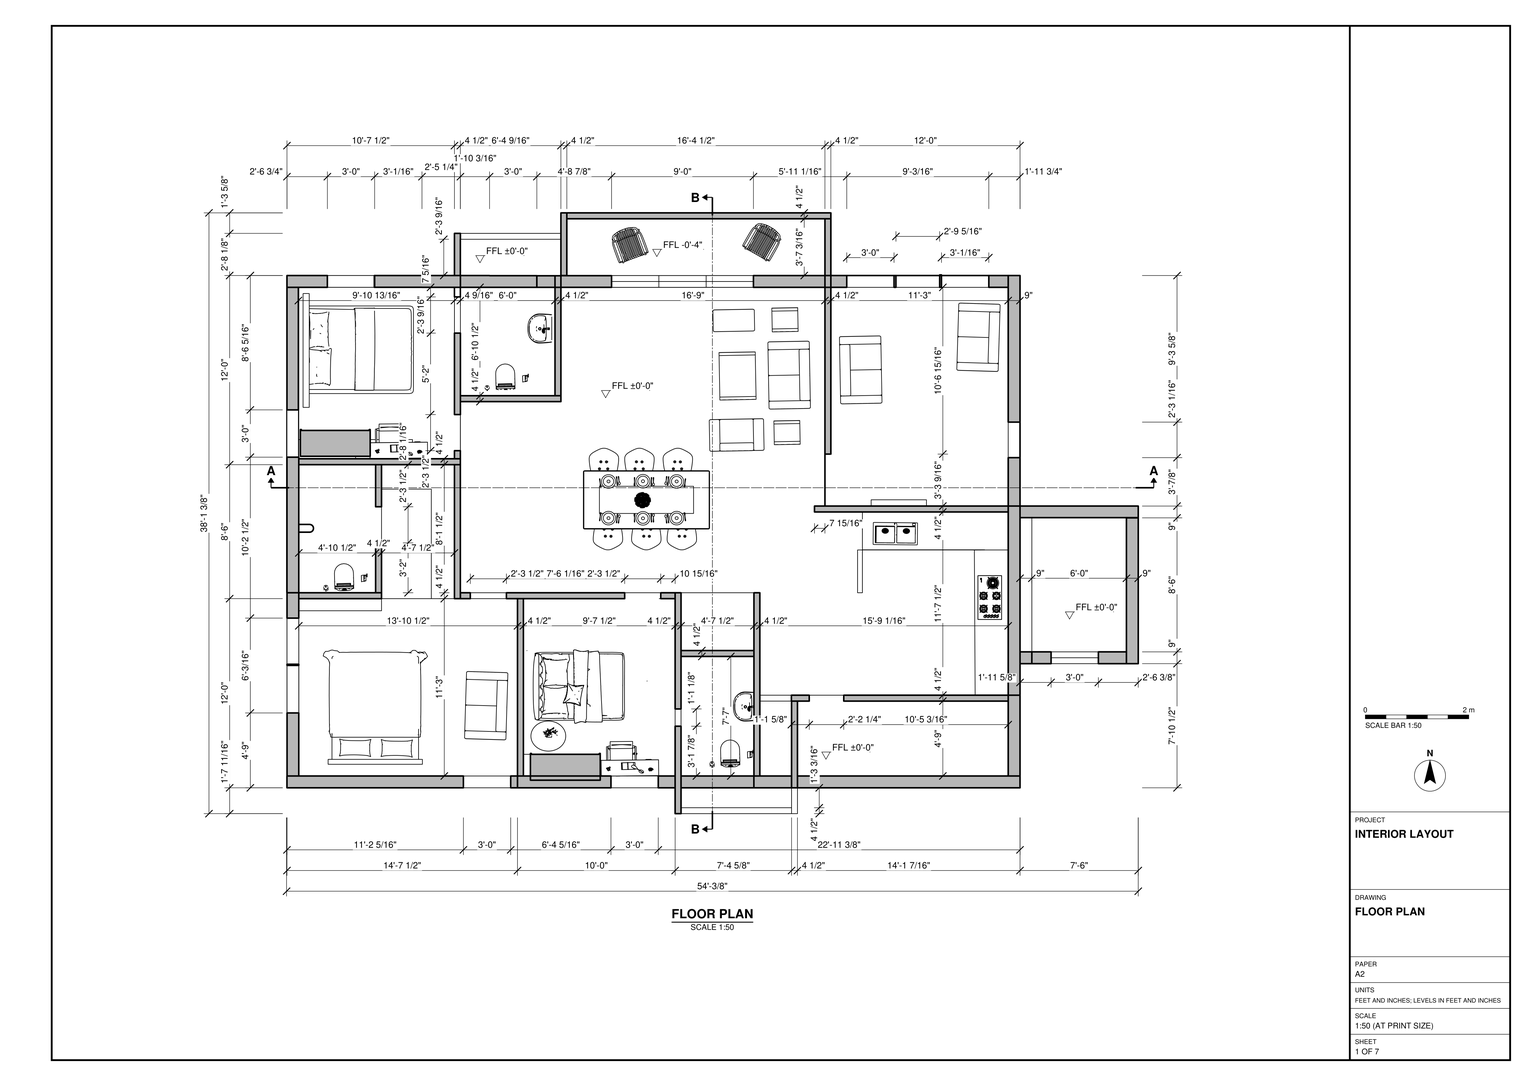
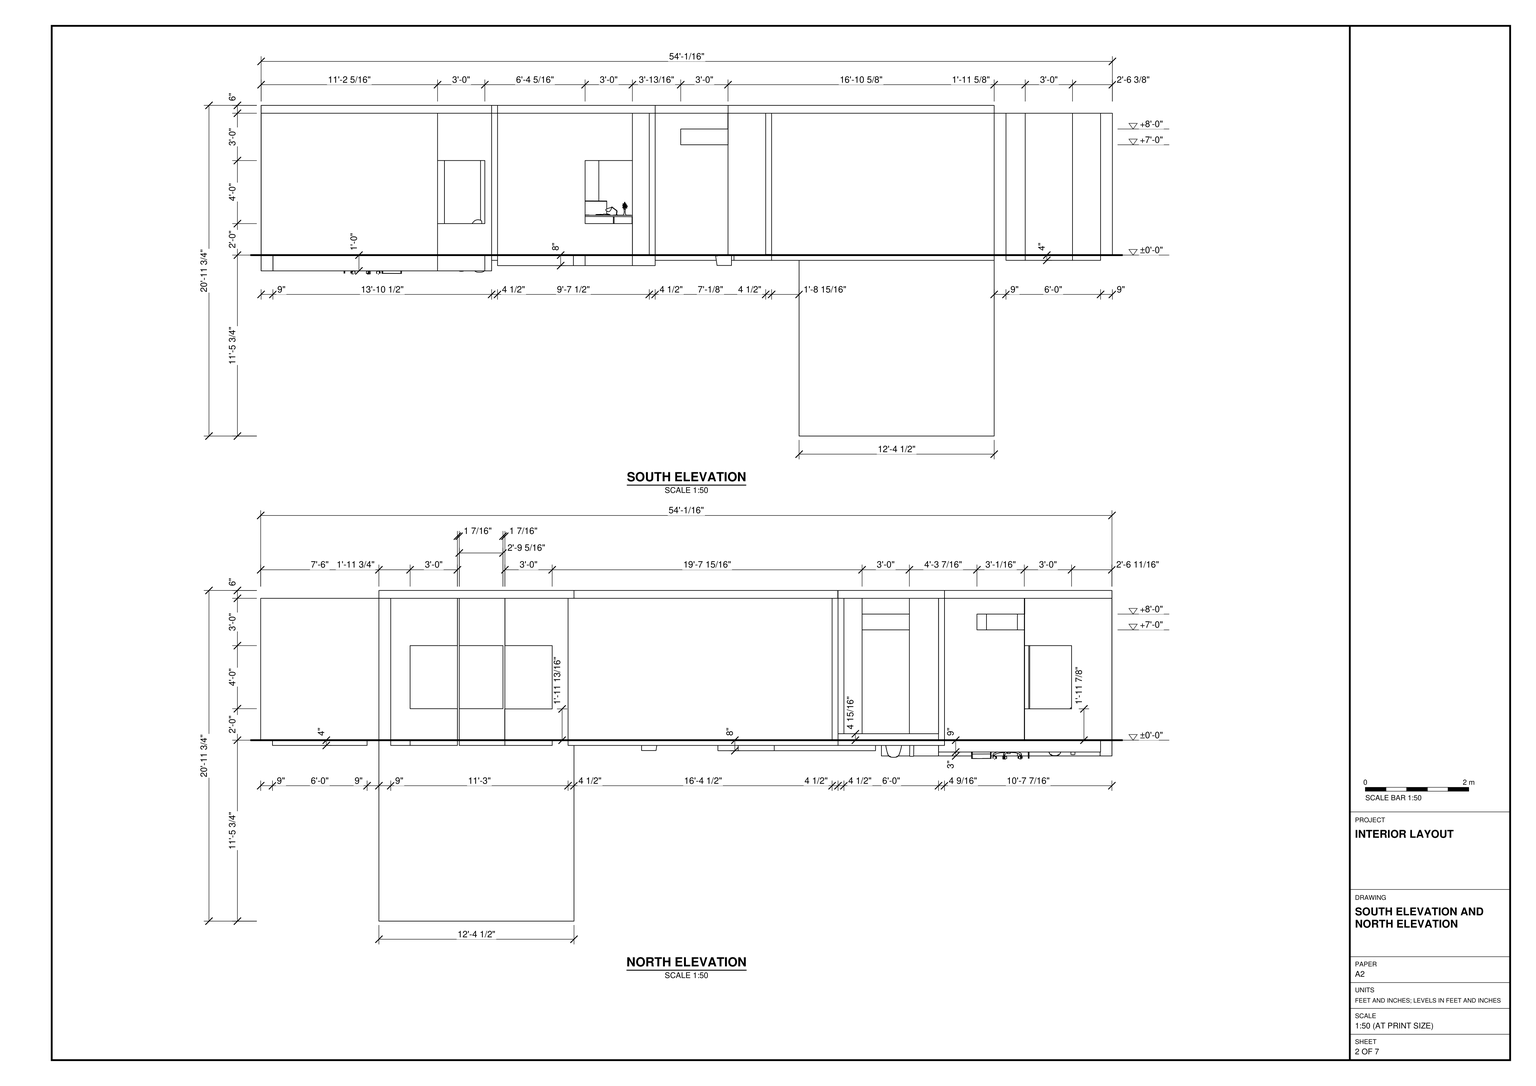
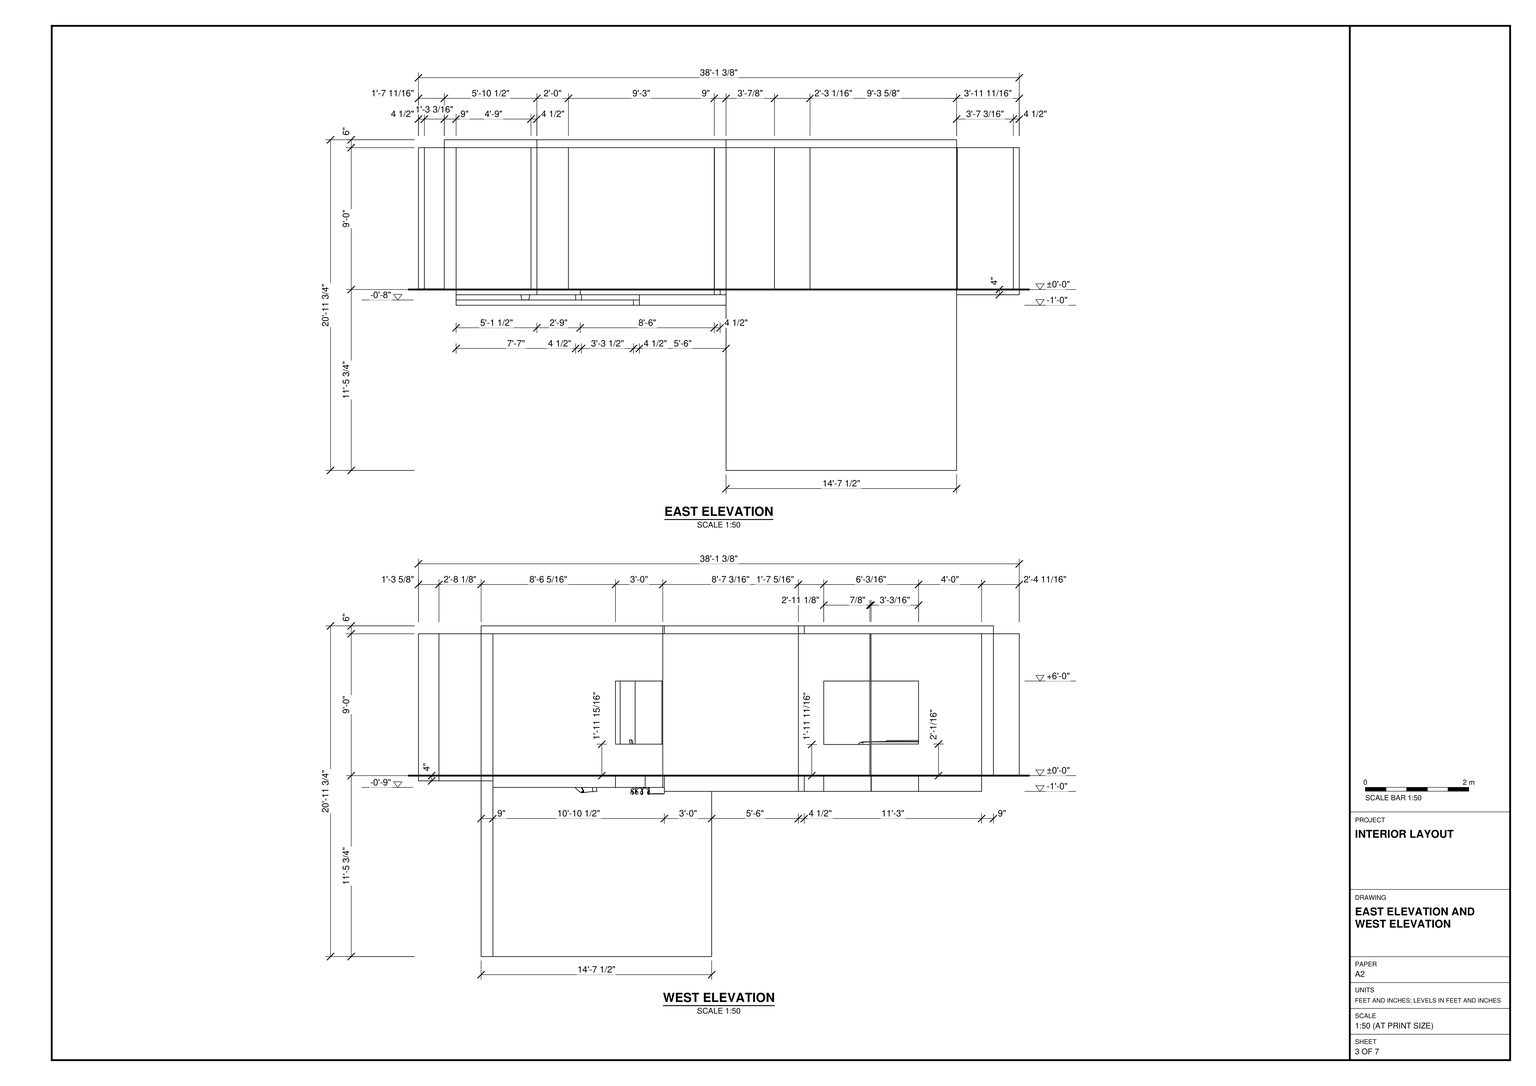
Build the interior shown in task_files/diagram_01.pdf in SketchUp. Work in feet and inches, with the main finished floor at ±0'-0". The overall model measures 54'-3/8" east to west, 38'-1 3/8" north to south and 20'-11 3/4" from bottom to top. The last dimension includes the portion below the floor shown in the elevations; it is not the room height.

Lay out the floor slabs and walls from the plan, including the shallow terrace on the north and the projection on the east. Use 9" perimeter walls and 4 1/2" partitions where dimensioned. Use the elevations to set the window sills, opening heights and flat roof slab. Keep the passages between rooms open where shown.

Place the living and dining furniture in the central space, with a separate seating area to the northeast. Fit the kitchen counters, sink and cooktop against the walls shown. Furnish the three bedrooms with beds in their drawn positions and include the desks, storage and bathroom fixtures shown on the plan. Match the footprints of the main furniture and joinery so that the clearances between pieces follow the drawing. Decor and loose items may be any suitable library components.

Keep walls, slabs, the roof and each furniture or joinery piece in separate groups or components, and use components for repeated parts. Save one SketchUp model as output_files/furnished_single_storey_residential_interior.skp.

# SketchUp Ruby script. Lengths in inches.
U = 1.inch
M = Sketchup.active_model
def pt(a) = Geom::Point3d.new(a.map { |v| v * U })
def face(e, loops, mat)
  f = e.add_face(loops[0].map { |a| pt(a) })
  loops[1..].each { |l| e.add_face(l.map { |a| pt(a) }).erase! }
  f.material = f.back_material = mat if mat
  f
end
# faces: each face lists its corners as indices into pts; further lists are holes
def faces(e, pts, list, mat = nil) = list.each { |f| face(e, (f[0].is_a?(Array) ? f : [f]).map { |l| l.map { |i| pts[i] } }, mat) }
# xy, xz, yz: faces in a plane at the given z, y or x. An outline is a flat list of corners, or four numbers for a rectangle; further outlines are holes
def ring(l) = l.size == 4 ? [[l[0], l[1]], [l[2], l[1]], [l[2], l[3]], [l[0], l[3]]] : l.each_slice(2).to_a
def flat(e, list, mat, &to3) = list.each { |f| face(e, (f[0].is_a?(Array) ? f : [f]).map { |l| ring(l).map { |u, v| to3.(u, v) } }, mat) }
def xy(e, z, list, mat = nil) = flat(e, list, mat) { |x, y| [x, y, z] }
def xz(e, y, list, mat = nil) = flat(e, list, mat) { |x, z| [x, y, z] }
def yz(e, x, list, mat = nil) = flat(e, list, mat) { |y, z| [x, y, z] }
def lines(e, pts, list) = list.each { |a, b| e.add_line(pt(pts[a]), pt(pts[b])) }
# prism: a flat outline (further loops are holes) pulled along v
def prism(e, loops, v, mat = nil)
  f = face(e, loops, mat); d = Geom::Vector3d.new(v.map { |x| x * U })
  f.pushpull(f.normal.samedirection?(d) ? d.length : -d.length)
end
def box(e, o, s, mat = nil) = prism(e, [[o, [o[0] + s[0], o[1], o[2]], [o[0] + s[0], o[1] + s[1], o[2]], [o[0], o[1] + s[1], o[2]]]], [0, 0, s[2]], mat)
def at(x, y, z, deg = 0) = Geom::Transformation.translation(pt([x, y, z])) * Geom::Transformation.rotation(ORIGIN, Z_AXIS, deg.degrees)
def axes(o, x, y, z) = Geom::Transformation.new([*x, 0, *y, 0, *z, 0, *pt(o).to_a, 1])
def part(name) = M.definitions.add(name)
# library, detail: a bought-in or finely detailed component or shape, given as its bounding box
def library(name, o, s) = part(name).tap { |d| box(d.entities, o, s) }
def detail(e, o, s) = box(e.add_group.entities, o, s)
def put(e, d, t, mat = nil) = e.add_instance(d, t).tap { |i| i.material = mat if mat }
def group(e, t, mat = nil) = e.add_group.tap { |g| g.transformation = t; g.material = mat if mat }.entities
root = M.entities
M.materials.add("\#ebbony").color = [77, 52, 40]
M.materials.add("[Color A02]").color = [65, 53, 38]
M.materials.add("[Encaustic Tile Circular 02]").color = [187, 174, 162]
M.materials.add("[Field Square Tile]").color = [217, 201, 169]
M.materials.add("[Stone Marble]").color = [143, 138, 136]
M.materials.add("[Tile Ceramic Multi]").color = [165, 115, 84]
M.materials.add("[Wood Veneer 01]").color = [89, 74, 63]
c1 = part("*U7")
p = [[-20,-17,0],[-20,23,0],[-18.25,23,0],[-18.25,-17,0],[20,-17,0],[19.92,-14.49,0],
  [19.68,-11.99,0],[19.29,-9.5,0],[18.74,-7.05,0],[18.04,-4.64,0],[17.19,-2.28,0],[16.19,0.03,0],
  [15.05,2.27,0],[13.77,4.43,0],[12.36,6.51,0],[10.82,8.5,0],[9.16,10.38,0],[7.38,12.16,0],
  [5.5,13.82,0],[3.51,15.36,0],[1.43,16.77,0],[-0.73,18.05,0],[-2.97,19.19,0],[-5.28,20.19,0],
  [-7.64,21.04,0],[-10.05,21.74,0],[-12.5,22.29,0],[-14.99,22.68,0],[-17.49,22.92,0],[-20,-23,0],
  [20,-23,0]]
lines(c1.entities,p,[[0,1],[1,2],[2,3],[3,0],[4,5],[5,6],[6,7],[7,8],[8,9],[9,10],[10,11],[11,12],
  [12,13],[13,14],[14,15],[15,16],[16,17],[17,18],[18,19],[19,20],[20,21],[21,22],[22,23],[23,24],
  [24,25],[25,26],[26,27],[27,28],[28,1],[0,29],[4,30]])
c2 = part("Component\#1")
xy(c2.entities,0,[[0,0,0,29.53,70.87,29.53,70.87,0,69.88,0,69.88,0.98,0.98,0.98,0.98,0]],"[Wood Veneer 01]")
xy(c2.entities,77.76,[[0.98,0,69.88,0.98]])
xy(c2.entities,78.74,[[0,0,70.87,29.53]],"[Wood Veneer 01]")
xz(c2.entities,0,[[0,0,0.98,0,0.98,77.76,69.88,77.76,69.88,0,70.87,0,70.87,78.74,0,78.74]],"[Wood Veneer 01]")
xz(c2.entities,0.98,[[0.98,0.98,69.88,77.76]])
xz(c2.entities,0.98,[[0.98,0,69.88,0.98]],"[Wood Veneer 01]")
xz(c2.entities,29.53,[[0,0,70.87,78.74]],"[Wood Veneer 01]")
yz(c2.entities,0,[[0,0,29.53,78.74]],"[Wood Veneer 01]")
yz(c2.entities,0.98,[[0,0,0.98,0.98],[0,0.98,0.98,77.76]],"[Wood Veneer 01]")
yz(c2.entities,69.88,[[0,0,0.98,0.98],[0,0.98,0.98,77.76]],"[Wood Veneer 01]")
yz(c2.entities,70.87,[[0,0,29.53,78.74]],"[Wood Veneer 01]")
c3 = library("Study desk set",[0,0,0],[44.11,35.83,41.8125])
c4 = library("Dining table set",[0,6.02,0],[90.69,75.24,42.02])
c5 = library("Cooktop+Brastemp+Ative!",[2.49,1.09,0.39],[33.46,18.11,1.98])
c6 = library("Double kitchen sink",[0,0,0],[33.74,16.9,23.42])
c7 = library("1.FBX",[-59.52,-60.59,0],[119.07,121.18,41.92])
c8 = library("Kohler_lavatory_wellworth_sink",[0,0,-7.24],[22.26,18.23,19.81])
c9 = library("Group\#63",[0,0,-0.01],[87.15,98.53,46.62])
c10 = library("Group\#114",[0,0,0],[41.34,31.5,26.77])
c11 = library("Group\#190",[11.8125,0,0],[21.65,31.5,16.93])
c12 = part("Group\#106")
xy(c12.entities,0.39,[[-1.57,1.38,18.11,19.09]])
xz(c12.entities,1.38,[[-1.57,0,18.11,0.39]])
xz(c12.entities,19.09,[[-1.57,0,18.11,0.39]])
yz(c12.entities,-1.57,[[1.38,0,19.09,0.39]])
yz(c12.entities,18.11,[[1.38,0,19.09,0.39]])
c13 = part("Group\#99")
xy(c13.entities,0,[[0,0,16.54,22.05]])
xy(c13.entities,1.18,[[0,0,16.54,22.05]])
xz(c13.entities,0,[[0,0,16.54,1.18]],"\#ebbony")
xz(c13.entities,22.05,[[0,0,16.54,1.18]],"\#ebbony")
yz(c13.entities,0,[[0,0,22.05,1.18]],"\#ebbony")
yz(c13.entities,16.54,[[0,0,22.05,1.18]],"\#ebbony")
c14 = library("Group\#193",[0,0,0],[31.5,66.93,26.77])
c15 = library("Group\#72",[0,0,0],[85.42,91.57,39.37])
c16 = library("Group\#85",[0,0,0],[23.58,22.35,32.36])
c17 = library("Group\#107",[0,0,0],[33.36,19.5,40.28])
box(root,[180.31,28.669,-8],[57.75,16.492,8])
xy(root,0,[[0.31,28.669,0.388,28.669,0.388,112.67,9.31,112.67,9.31,112.853,0.36,112.853,0.36,163.669,0.31,163.669],[360.31,28.669,384.3125,85.672],[0.388,76.67,4.888,112.67],[4.888,76.67,9.31,112.67],[9.31,76.67,9.388,112.67],
  [434.698,85.672,531.416,90.172],[531.416,90.172,532.014,90.172,531.416,200.737],[9.31,112.853,9.36,148.853],[0.36,113.728,4.86,148.853],[4.86,113.728,9.31,148.853],
  [567.365,114.172,582.002,123.172],[0.31,163.669,0.36,168.169],[132.31,163.669,132.365,168.169],[0,168.169,0.31,271.379],[434.698,168.169,438.365,200.737],
  [438.365,200.737,531.416,200.737,531.415,200.881,438.365,200.881],[445.036,234.172,487.134,238.932],[9,270.169,9.31,307.379],[132.31,270.169,132.365,303.816],[0,271.379,0.31,307.379],
  [132.31,303.816,132.365,307.379],[132.31,307.379,132.365,318.172],[132.365,400.548,154.538,400.672],[154.538,400.548,190.538,400.672],[247.424,400.628,283.424,400.672],
  [283.424,400.628,319.424,400.672],[319.424,400.628,355.424,400.672],[66.82,400.672,67.102,400.672,67.102,409.669,67.07,409.669,67.07,400.705,66.82,400.705],[498.573,400.672,498.614,409.672],[208.865,409.548,247.424,409.628],
  [31.07,409.669,67.07,409.705],[67.105,409.669,103.105,409.705],[127.81,409.669,132.31,409.672],[132.31,409.672,132.365,437.265]])
xy(root,108,[[175.81,19.669,180.31,163.669],[208.865,233.549,209.053,400.672],[355.81,233.549,409.865,234.172],[208.865,400.672,409.865,452.877]])
p = [[67.81,233.63,0],[67.81,233.633,0],[31.07,405.205,0],[66.82,405.205,0],[67.105,405.205,0],[67.105,409.669,0],
  [103.105,400.705,0],[67.105,400.705,0],[103.105,405.205,0],[4.5,307.379,0],[4.5,271.379,0],[154.538,409.548,0],
  [190.538,409.548,0],[154.538,405.048,0],[190.538,405.048,0],[247.424,409.628,0],[283.424,409.628,0],[283.424,405.128,0],
  [247.424,405.128,0],[319.424,409.628,0],[319.424,405.128,0],[355.424,409.628,0],[355.424,405.128,0],[426.456,405.172,0],
  [462.456,405.172,0],[498.614,405.172,0],[534.614,405.172,0],[582.002,118.672,0],[618.002,118.672,0],[283.685,163.669,0],
  [284.887,163.669,0],[9.31,400.669,0],[127.81,400.669,0],[246.967,24.169,0],[282.967,24.169,0],[134.637,24.169,0],
  [170.637,24.169,0],[9.36,154.461,0],[72.31,154.461,0],[618.002,114.172,0],[582.002,114.172,0],[283.424,400.672,0],
  [319.424,400.672,0],[72.31,163.669,0],[67.81,206.151,0],[67.81,207.353,0],[127.81,393.387,0],[127.81,365.84,0],
  [295.81,79.705,0],[295.81,66.571,0],[424.187,85.672,0],[424.184,85.672,0],[355.764,19.669,0],[319.764,19.669,0],
  [282.967,19.669,0],[246.967,19.669,0],[170.637,19.669,0],[134.637,19.669,0],[132.31,393.387,0],[132.31,392.11,0],
  [426.456,409.672,0],[462.456,409.672,0],[558.365,298.068,0],[558.365,271.022,0],[498.614,409.672,0],[534.614,409.672,0],
  [9.31,307.379,0],[648.365,225.348,0],[648.365,225.172,0],[497.198,400.672,0],[462.573,400.672,0],[66.82,400.705,0],
  [31.07,400.705,0],[67.102,409.669,0]]
lines(root,p,[[0,1],[2,3],[4,5],[6,7],[7,4],[4,8],[9,10],[11,12],[13,14],[15,16],[16,17],[18,17],
  [16,19],[19,20],[19,21],[20,22],[23,24],[25,26],[27,28],[29,30],[31,32],[33,34],[35,36],[37,38],
  [39,40],[41,17],[42,20],[43,38],[44,45],[46,47],[48,49],[50,51],[52,53],[54,55],[56,57],[58,59],
  [60,61],[62,63],[64,65],[66,31],[17,20],[67,68],[69,70],[71,72],[73,5]])
put(root,c1,axes([56.51,219.89,0],[0,0.68705,0],[-0.68705,0,0],[0,0,0.68705]))
put(root,c1,axes([153.625,152.37,0],[-0.68705,0,0],[0,-0.68705,0],[0,0,0.68705]))
put(root,c1,axes([271.15,152.4375,0],[-0.68705,0,0],[0,-0.68705,0],[0,0,0.68705]))
put(root,c1,axes([410.45,74.37,0],[0.68705,0,0],[0,-0.68705,0],[0,0,0.68705]))
put(root,c1,axes([303.5,73.26,0],[0,0.33421,0],[0.33421,0,0],[0,0,0.33421]))
put(root,c1,axes([542.5625,284.76,0],[0,0.68705,0],[-0.68705,0,0],[0,0,0.68705]))
put(root,c1,axes([143.4,379.4,0],[-0.01076,-0.68696,0],[0.68696,-0.01076,0],[0,0,0.68705]))
put(root,c2,axes([63.67,292.42,12],[-0.75,0,0],[0,-0.69,0],[0,0,1.23]),"[Color A02]")
put(root,c3,axes([63.5,270.17,-14.18],[0.99173,0.01039,-0.00502],[-0.00767,0.72995,-0.00408],[0.00501,0.00565,0.99997]))
put(root,c4,axes([322.07,284.38,0],[-1.06,0,0],[0,-1.0282,0],[0,0,0.689]))
put(root,c5,at(525.19,183.73,31.37,-90))
put(root,c6,axes([446.55,204.375,22.5],[0.99988,-0.01203,0.00943],[0.01249,0.99866,-0.05015],[-0.00881,0.05026,0.9987]))
put(root,c7,axes([228.78,85.92,0.14],[0.00004,0.65328,0.00643],[-0.75684,-0.00005,0.00967],[0.01277,-0.00985,0.99987]))
put(root,c2,axes([238.8,45.84,0],[-0.75,0,0],[0,-0.69,0],[0,0,1.23]),"[Color A02]")
put(root,c3,axes([239.42,28.36,-0.33],[0.99173,0.01039,-0.00502],[-0.00767,0.72995,-0.00408],[0.00501,0.00565,0.99997]))
put(root,c8,axes([27.54,205.875,53.12],[-0.00001,1,0],[-1,-0.00001,-0.00002],[-0.00002,0,1]))
put(root,c8,axes([183.68,380.47,34.06],[0.00001,-1,0],[1,0.00001,-0.00002],[0.00002,0,1]))
put(root,c8,axes([340.17,92.67,-0.63],[0.00001,-1,0],[1,0.00001,-0.00002],[0.00002,0,1]))
g1 = group(root,at(0.31,19.67,0))
prism(g1,[[[0,0,0],[0,9,0],[0.08,9,0],[9,9,0],[134.33,9,0],[134.33,0,0]]],[0,0,108])
g2 = group(root,at(0.39,28.67,0))
prism(g2,[[[0,84.18,0],[0,0,0],[0,0,108],[0,84.25,108],[0,84.25,72],[0,48,72],[0,48,24.0625],[0,84.18,24.0625]]],[8.92,0,0])
g3 = group(root,at(170.64,19.67,0))
prism(g3,[[[5.17,9,0],[-36,9,0],[-36,9,24],[0,9,24],[0,9,72],[-36,9,72],[-36,9,108],[5.17,9,108]]],[0,-9,0])
g4 = group(root,at(0.36,148.85,0))
xy(g4,0,[[0,-35.125,8.95,19.32]])
xy(g4,23.6875,[[0,-35.125,8.95,0]])
xy(g4,72,[[0,-35.125,8.95,0]])
xy(g4,108,[[0,-35.125,8.95,19.32]])
xz(g4,-35.125,[[0,0,8.95,23.6875],[0,72,8.95,108]])
xz(g4,0,[[0,23.6875,8.95,72]])
xz(g4,19.32,[[0,0,8.95,108]])
yz(g4,0,[[-35.125,0,-35.125,23.6875,0,23.6875,0,72,-35.125,72,-35.125,108,19.32,108,19.32,0]])
yz(g4,8.95,[[-35.125,0,14.82,0,14.82,108,-35.125,108,-35.125,72,0,72,0,23.6875,-35.125,23.6875],[14.82,0,19.32,108]])
g5 = group(root,at(175.81,19.67,0))
xy(g5,0,[[0,0,107.22,9]])
xy(g5,24,[[71.16,0,107.22,9]])
xy(g5,72,[[71.16,0,107.16,9]])
xy(g5,108,[[0,0,107.16,9]])
xz(g5,0,[[0,0,4.5,108],[4.5,0,107.22,0,107.22,24,71.16,24,71.16,72,107.16,72,107.16,108,4.5,108]])
xz(g5,9,[[0,0,4.5,108],[4.5,0,62.25,108],[62.25,0,62.25,108,107.16,108,107.16,72,71.16,72,71.16,24,107.22,24,107.22,0]])
yz(g5,0,[[0,0,9,108]])
yz(g5,71.16,[[0,24,9,72]])
yz(g5,107.16,[[0,72,9,108]])
yz(g5,107.22,[[0,0,9,24]])
g6 = group(root,at(175.81,28.67,0))
prism(g6,[[[4.5,135,0],[4.5,16.49,0],[4.5,0,0],[0,0,0],[0,37.71,0],[0,135,0]]],[0,0,108])
g7 = group(root,at(282.97,19.67,0))
box(g7,[0,0,0],[12.84,9,108])
g8 = group(root,at(167.37,163.67,0))
prism(g8,[[[90.04,0,0],[12.94,0,0],[8.44,0,0],[0,0,0],[0,4.5,0],[90.04,4.5,0]]],[0,0,108])
g9 = group(root,at(284.89,163.67,0))
box(g9,[0,0,0],[10.92,4.5,108])
g10 = group(root,at(295.81,79.71,0))
prism(g10,[[[0,88.46,0],[4.5,88.46,0],[4.5,83.96,0],[4.5,44.46,0],[4.5,39.96,0],[4.5,0,0],[0,0,0],[0,83.96,0]]],[0,0,108])
g11 = group(root,at(295.81,0,0))
prism(g11,[[[4.5,0,0],[0,0,0],[0,19.67,0],[0,28.67,0],[0,66.57,0],[4.5,66.57,0],[4.5,28.67,0],[4.5,19.67,0],[4.5,4.5,0]]],[0,0,108])
g12 = group(root,at(300.31,0,0))
xy(g12,0,[[0,0,84.14,4.5]])
g13 = group(root,at(355.76,19.67,0))
prism(g13,[[[28.68,0,0],[0,0,0],[0,9,0],[0.05,9,0],[4.55,9,0],[28.68,9,0]]],[0,0,108])
g14 = group(root,at(355.81,28.67,0))
prism(g14,[[[4.5,0,0],[0,0,0],[0,91,0],[0,95.5,0],[0,139.5,0],[4.5,139.5,0],[4.5,61.5,0],[4.5,57,0]]],[0,0,108])
g15 = group(root,at(300.31,119.67,0))
box(g15,[0,0,0],[55.5,4.5,108])
g16 = group(root,at(384.45,0,0))
prism(g16,[[[0,85.67,0],[4.5,85.67,0],[4.5,28.67,0],[4.5,19.67,0],[4.5,0,0],[0,0,0],[0,4.5,0],[0,19.67,0],[0,28.67,0]]],[0,0,0.5])
g17 = group(root,at(424.1875,85.67,0))
prism(g17,[[[125.18,4.5,0],[125.18,0,0],[21.02,0,0],[0,0,0],[0,4.5,0],[107.83,4.5,0]]],[0,0,108])
g18 = group(root,at(388.95,19.67,0))
prism(g18,[[[169.42,0,0],[0,0,0],[0,9,0],[160.42,9,0],[169.42,9,0]]],[0,0,108])
g19 = group(root,at(549.37,28.67,0))
prism(g19,[[[9,0,0],[0,0,0],[0,57,0],[0,61.5,0],[9,61.5,0],[9,57,0]]],[0,0,108])
g20 = group(root,at(549.37,90.17,0))
prism(g20,[[[9,0,0],[0,0,0],[0,139.5,0],[0,144,0],[9,144,0],[9,139.5,0],[9,24,0]]],[0,0,108])
g21 = group(root,at(401.9,229.67,0))
prism(g21,[[[85.23,4.5,0],[147.46,4.5,0],[147.46,0,0],[36.46,0,0],[0,0,0],[0,4.5,0],[7.96,4.5,0],[12.46,4.5,0],[43.13,4.5,0]]],[0,0,108])
g22 = group(root,at(300.31,19.67,0))
prism(g22,[[[0,0,0],[55.45,0,0],[55.45,0,84],[19.45,0,84],[19.45,0,96],[55.33,0,96],[55.33,0,108],[0,0,108]]],[0,9,0])
g23 = group(root,at(9.31,163.67,0))
prism(g23,[[[0,4.5,0],[58.5,4.5,0],[63,4.5,0],[63,0,0],[0,0,0]]],[0,0,108])
g24 = group(root,at(67.81,168.17,0))
box(g24,[0,0,0],[4.5,37.98,108])
g25 = group(root,at(67.81,233.63,0))
prism(g25,[[[0,32.04,0],[4.5,32.04,0],[4.5,13.41,0],[4.5,0,0],[0,0,0]]],[0,0,108])
g26 = group(root,at(9.31,265.67,0))
prism(g26,[[[0,0,0],[0,4.5,0],[43.27,4.5,0],[63,4.5,0],[86.53,4.5,0],[118.5,4.5,0],[123,4.5,0],[123,0,0],[118.5,0,0],[63,0,0],[58.5,0,0]]],[0,0,108])
g27 = group(root,at(0.31,168.17,0))
prism(g27,[[[9,102,0],[9,0,0],[0.05,0,0],[0,0,0],[0,103.21,0],[8.69,103.21,0],[9,103.21,0]]],[0,0,108])
g28 = group(root,at(0.31,307.38,0))
prism(g28,[[[0,93.29,0],[0,-36,0],[0,-36,23.9375],[0,0,23.9375],[0,0,72],[0,-36,72],[0,-36,108],[0,93.29,108]]],[8.69,0,0])
g29 = group(root,at(0.31,400.67,0))
xy(g29,0,[[0,0,0,9,66.51,9,66.51,0.03,30.76,0.03,30.76,0]])
xy(g29,23.875,[[30.76,0.03,66.51,9]])
xy(g29,72,[[30.76,0.03,66.51,9]])
xy(g29,108,[[0,0,30.76,0,30.76,0.03,66.51,0.03,66.51,9,0,9]])
xz(g29,0,[[0,0,8.69,108],[8.69,0,30.76,108]])
xz(g29,0.03,[[30.76,0,66.51,23.875],[30.76,72,66.51,108]])
xz(g29,9,[[0,0,0,108,66.51,108,66.51,72,30.76,72,30.76,23.875,66.51,23.875,66.51,0]])
yz(g29,0,[[0,0,9,108]])
yz(g29,30.76,[[0,0,0.03,108],[0.03,23.875,9,72]])
yz(g29,66.51,[[0.03,0,9,23.875],[0.03,72,9,108]])
g30 = group(root,at(103.1,400.67,0))
xy(g30,0,[[0,0,0,0.03,-36.03,0.03,-36.03,9,29.26,9,29.26,0]])
xy(g30,84,[[-36.03,0.03,0,9]])
xy(g30,96,[[-36.375,0.03,0,9]])
xy(g30,108,[[0,0,29.26,0,29.26,9,-36.375,9,-36.375,0.03,0,0.03]])
xz(g30,0,[[0,0,29.26,108]])
xz(g30,0.03,[[-36.03,0,0,84],[-36.375,96,0,108]])
xz(g30,9,[[-36.03,0,-36.03,84,0,84,0,96,-36.375,96,-36.375,108,24.71,108,24.71,0],[24.71,0,29.21,108],[29.21,0,29.26,108]])
yz(g30,-36.375,[[0.03,96,9,108]])
yz(g30,-36.03,[[0.03,0,9,84]])
yz(g30,0,[[0,0,0.03,108],[0.03,84,9,96]])
yz(g30,29.26,[[0,0,9,108]])
p = [[0,9,72],[0,9.03,72],[0,9,23.875],[0,9.03,23.875]]
lines(g30,p,[[0,1],[2,3]])
g31 = group(root,at(132.37,400.67,0))
xy(g31,0,[[0,0,0,9,22.17,9,22.17,8.875,58.17,8.875,58.17,0]])
xy(g31,84,[[22.17,0,58.17,8.875]])
xy(g31,96,[[22.17,0,58.17,8.875]])
xy(g31,108,[[0,0,58.17,0,58.17,8.875,22.17,8.875,22.17,9,0,9]])
xz(g31,0,[[0,0,58.17,0,58.17,84,22.17,84,22.17,96,58.17,96,58.17,108,0,108]])
xz(g31,8.875,[[22.17,0,58.17,84],[22.17,96,58.17,108]])
xz(g31,9,[[0,0,22.17,108]])
yz(g31,0,[[0,0,9,108]])
yz(g31,22.17,[[8.875,0,9,108],[0,84,8.875,96]])
yz(g31,58.17,[[0,0,8.875,84],[0,96,8.875,108]])
p = [[22.17,0,84],[22.17,-0.0625,84]]
lines(g31,p,[[0,1]])
g32 = group(root,at(127.81,270.17,0))
box(g32,[0,0,0],[4.5,6.17,108])
g33 = group(root,at(127.81,303.82,0))
prism(g33,[[[4.56,0,0],[4.5,0,0],[0,0,0],[0,62.02,0],[4.56,62.02,0],[4.56,14.36,0],[4.56,9.86,0]]],[0,0,108])
g34 = group(root,at(127.81,393.39,0))
box(g34,[0,0,0],[4.5,7.28,108])
g35 = group(root,at(132.37,313.67,0))
prism(g35,[[[76.5,4.5,0],[76.5,0,0],[0,0,0],[0,4.5,0],[72,4.5,0]]],[0,0,108])
g36 = group(root,at(204.37,318.17,0))
box(g36,[0,0,0],[4.5,82.5,108])
g37 = group(root,at(132.37,437.26,0))
box(g37,[0,0,0],[76.5,4.5,4.9375])
g38 = group(root,at(127.81,409.67,0))
prism(g38,[[[4.56,27.59,0],[4.5,27.59,0],[4.5,0,0],[0,0,0],[0,32.09,0],[4.56,32.09,0]]],[0,0,108])
g39 = group(root,at(208.87,409.67,0))
prism(g39,[[[4.5,0,0],[0,0,0],[0,27.59,0],[0,32.09,0],[0,47.7,0],[4.5,47.7,0],[4.5,43.2,0],[4.5,32.09,0]]],[0,0,108])
g40 = group(root,at(213.37,452.88,0))
prism(g40,[[[201,4.5,0],[201,0,0],[196.5,0,0],[0,0,0],[0,4.5,0]]],[0,0,108])
g41 = group(root,at(409.87,409.67,0))
box(g41,[0,0,0],[4.5,43.2,108])
g42 = group(root,at(355.42,400.67,0))
prism(g42,[[[58.94,0,0],[54.44,0,0],[0,0,0],[0,4.46,0],[0,8.96,0],[58.94,8.96,0]]],[0,0,108])
g43 = group(root,at(409.87,273.72,0))
box(g43,[0,0,0],[4.5,126.95,108])
g44 = group(root,at(190.54,400.67,0))
box(g44,[13.83,0,0],[4.5,8.8125,108])
p = [[18.33,0,0],[56.89,0,0],[41.1875,8.875,0],[56.89,8.875,0]]
lines(g44,p,[[0,1],[2,3],[3,1]])
g45 = group(root,at(208.87,400.67,0))
prism(g45,[[[22.86,0,0],[0,0,0],[0,8.875,0],[22.86,8.875,0],[38.56,8.875,0],[38.56,4.46,0],[38.56,0,0]]],[0,0,108])
g46 = group(root,at(414.37,400.67,0))
prism(g46,[[[0,0,0],[48.09,0,0],[48.09,0,23.8125],[12.09,0,23.8125],[12.09,0,72],[48.03,0,72],[48.03,0,108],[0,0,108]]],[0,9,0])
g47 = group(root,at(534.61,400.67,0))
prism(g47,[[[14.75,9,0],[-36,9,0],[-36,9,24],[0,9,24],[0,9,72],[-36,9,72],[-36,9,108],[14.75,9,108]]],[0,-9,0])
g48 = group(root,at(549.37,298.07,0))
prism(g48,[[[9,0,0],[0,0,0],[0,102.6,0],[0,111.6,0],[9,111.6,0]]],[0,0,108])
g49 = group(root,at(549.37,234.17,0))
box(g49,[0,0,0],[9,36.85,108])
g50 = group(root,at(360.31,85.67,0))
xy(g50,0,[[0,0,37.6,4.5]])
g51 = group(root,at(384.45,19.67,0.5))
box(g51,[0,0,0],[4.5,66,107.5])
g52 = group(root,at(384.3125,85.67,0))
prism(g52,[[[13.6,4.5,0],[13.6,0,0],[0,0,0],[0,4.5,0],[4.64,4.5,0]]],[0,0,108])
put(root,c9,axes([12.58,309.26,0],[0.96444,0,0],[0,0.8802,0],[0,0,0.92]))
g53 = group(root,at(190.54,400.67,0))
box(g53,[0,0,0],[13.83,8.8125,108])
g54 = group(root,at(132.37,163.67,0))
box(g54,[0,0,0],[7.52,4.5,108])
g55 = group(root,at(127.81,163.67,0))
prism(g55,[[[4.5,0,0],[0,0,0],[0,102,0],[4.5,102,0],[4.5,4.5,0]]],[0,0,108])
g56 = group(root,at(398.8,275.84,0,90))
put(g56,c10,axes([0.09,76.61,-0.01],[0.0182,-0.99983,-0.00006],[0.76426,0.01391,0.00449],[-0.00587,-0.00017,0.99998]))
put(g56,c11,axes([82.11,73.78,0.48],[0.76426,0.01391,0.00449],[0.0182,-0.99983,-0.00006],[-0.00587,-0.00017,0.99998]))
g57 = group(g56,at(39.11,68.93,0.22))
p = [[0,0,0],[0.5,-27.55,0],[0.42,-27.56,13.78],[-0.08,0,13.78],[0.01,-0.79,0.79],[-0.0625,-0.79,12.99],
  [0.41,-26.77,12.99],[0.48,-26.77,0.79],[4.51,0.08,0.03],[5.02,-27.47,0.02],[4.9375,-27.47,13.41],[2.68,-27.52,13.4],
  [2.68,-27.52,13.79],[4.43,0.08,13.41],[4.45,-0.71,13.02],[4.52,-0.71,0.8125],[5,-26.69,0.8125],[4.92,-26.6875,13.02],
  [2.18,0.04,13.79],[2.18,0.04,13.4],[32.02,-26.98,13.57],[31.51,0.57,13.57],[31.59,0.58,0.1875],[32.1,-26.98,0.18],
  [31.6,-0.21,0.97],[31.53,-0.21,13.18],[32,-26.19,13.18],[32.08,-26.19,0.97],[36.11,0.66,0.21],[36.61,-26.9,0.21],
  [36.53,-26.9,13.99],[34.27,-26.94,13.98],[34.27,-26.94,13.58],[36.03,0.65,13.99],[36.04,-0.13,13.2],[36.12,-0.13,1],
  [36.59,-26.11,1],[36.52,-26.11,13.2],[33.77,0.61,13.58],[33.77,0.61,13.98],[1.07,-25.97,1.58],[0.62,-1.5625,1.58],
  [1,-25.97,12.21],[3.93,-1.5,1.6],[4.375,-25.91,1.6],[4.3125,-25.91,12.23],[0.56,-1.57,12.21],[3.87,-1.51,12.23],
  [32.66,-25.39,1.76],[32.21,-0.99,1.76],[32.6,-25.4,12.39],[35.52,-0.93,1.78],[35.97,-25.33,1.78],[35.91,-25.34,12.41],
  [32.15,-0.99,12.39],[35.46,-0.93,12.41]]
faces(g57,p,[[[0,1,2,3],[4,5,6,7]],[1,0,8,9],[9,10,11,12,2,1],[[8,13,10,9],[14,15,16,17]],[3,18,19,13,8,0],[[20,21,22,23],[24,25,26,27]],[28,29,23,22],[30,31,32,20,23,29],
  [[29,28,33,30],[34,35,36,37]],[22,21,38,39,33,28],[4,7,40,41],[7,6,42,40],[16,15,43,44],[17,16,44,45],[5,4,41,46],[15,14,47,43],
  [24,27,48,49],[27,26,50,48],[36,35,51,52],[37,36,52,53],[25,24,49,54],[35,34,55,51],[41,40,44,43],[42,45,44,40],
  [41,43,47,46],[49,48,52,51],[50,53,52,48],[49,51,55,54],[6,5,46,42],[14,17,45,47],[47,45,42,46],[26,25,54,50],
  [34,37,53,55],[55,53,50,54],[12,11,19,18],[11,10,13,19],[20,32,38,21],[32,31,39,38],[12,18,3,2],[33,39,31,30]],"\#ebbony")
g58 = group(g57,at(0.59,-1.56,6.3),"\#ebbony")
p = [[0.4375,-24.41,1.18],[-0.01,0,1.18],[0,0,0],[0.44,-24.41,0],[35.35,-23.77,0.2],[34.9,0.64,0.2],
  [35.34,-23.77,1.38],[34.9,0.64,1.39]]
faces(g58,p,[[0,1,2,3],[6,0,3,4],[1,7,5,2],[7,6,4,5]],"\#ebbony")
faces(g58,p,[[4,3,2,5],[0,6,7,1]])
g59 = group(g57,at(1.15,-1.55,13.39))
p = [[1.52,-25.96,0.4],[1.02,1.59,0.4],[1.02,1.59,0.01],[1.53,-25.96,0],[33.12,-25.39,0.19],[33.12,-25.39,0.58],
  [32.62,2.17,0.59],[32.62,2.17,0.19]]
faces(g59,p,[[0,1,2,3],[3,4,5,0],[1,6,7,2],[6,5,4,7],[1,0,5,6]])
g60 = group(g56,at(5.1,27.48,0.02))
xy(g60,13.4,[[2.54,-19.64,3.29,-19.63,2.93,0.05,2.18,0.04]],"\#ebbony")
p = [[-0.08,0,13.78],[0,0,0],[0.36,-19.68,0],[0.28,-19.68,13.78],[0.01,-0.79,0.79],[-0.0625,-0.79,12.99],
  [0.27,-18.9,12.99],[0.34,-18.89,0.79],[3.37,-19.625,0.02],[3.01,0.05,0.02],[3.29,-19.63,13.4],[2.54,-19.64,13.4],
  [2.53,-19.64,13.79],[2.93,0.05,13.4],[3.02,-0.73,0.81],[3.35,-18.84,0.8],[3.28,-18.84,13.01],[2.95,-0.73,13.01],
  [2.18,0.04,13.79],[2.18,0.04,13.4],[15.32,-19.41,13.47],[14.97,0.27,13.47],[15.04,0.27,0.09],[15.4,-19.41,0.09],
  [14.98,-0.52,13.08],[15.3125,-18.62,13.08],[15.38,-18.62,0.875],[15.05,-0.51,0.875],[18.41,-19.35,0.1],[18.05,0.33,0.11],
  [18.33,-19.36,13.88],[16.07,-19.4,13.87],[16.08,-19.4,13.48],[17.97,0.33,13.89],[18.39,-18.57,0.89],[18.32,-18.57,13.1],
  [17.99,-0.46,13.1],[18.0625,-0.46,0.89],[15.72,0.29,13.87],[15.72,0.29,13.48],[0.62,-1.5625,1.58],[0.92,-18.1,1.58],
  [0.86,-18.1,12.21],[2.43,-1.53,1.59],[2.73,-18.0625,1.59],[2.67,-18.07,12.22],[0.56,-1.57,12.21],[2.36,-1.53,12.22],
  [15.67,-1.29,1.67],[15.97,-17.82,1.67],[15.9,-17.82,12.3],[17.47,-1.26,1.68],[17.77,-17.79,1.68],[17.71,-17.79,12.31],
  [15.6,-1.29,12.3],[17.41,-1.26,12.31]]
faces(g60,p,[[[0,1,2,3],[4,5,6,7]],[8,2,1,9],[8,10,11,12,3,2],[[8,9,13,10],[14,15,16,17]],[0,18,19,13,9,1],[[20,21,22,23],[24,25,26,27]],[28,23,22,29],[20,23,28,30,31,32],
  [[30,28,29,33],[34,35,36,37]],[38,33,29,22,21,39],[40,4,7,41],[7,6,42,41],[14,43,44,15],[16,15,44,45],[5,4,40,46],[14,17,47,43],
  [48,27,26,49],[26,25,50,49],[37,51,52,34],[35,34,52,53],[24,27,48,54],[37,36,55,51],[43,40,41,44],[42,45,44,41],
  [40,43,47,46],[51,48,49,52],[50,53,52,49],[48,51,55,54],[42,6,5,46],[16,45,47,17],[45,42,46,47],[50,25,24,54],
  [35,53,55,36],[53,50,54,55],[18,12,11,19],[39,21,20,32],[39,32,31,38],[18,0,3,12],[33,38,31,30]],"\#ebbony")
put(g60,c12,axes([1.15,-1.55,13.39],[0.0182,-0.99983,-0.00006],[0.76426,0.01391,0.00449],[-0.00587,-0.00017,0.99998]))
put(g60,c13,axes([0.59,-1.56,6.55],[0.0182,-0.99983,-0.00006],[0.76426,0.01391,0.00449],[-0.00587,-0.00017,0.99998]),"\#ebbony")
g61 = group(g56,at(90.99,29.05,0.52))
xy(g61,13.4,[[2.54,-19.64,3.29,-19.63,2.93,0.05,2.18,0.04]],"\#ebbony")
p = [[-0.08,0,13.78],[0,0,0],[0.36,-19.68,0],[0.28,-19.68,13.78],[0.01,-0.79,0.79],[-0.0625,-0.79,12.99],
  [0.27,-18.9,12.99],[0.34,-18.89,0.79],[3.37,-19.625,0.02],[3.01,0.05,0.02],[3.29,-19.63,13.4],[2.54,-19.64,13.4],
  [2.53,-19.64,13.79],[2.93,0.05,13.4],[3.02,-0.73,0.81],[3.35,-18.84,0.8],[3.28,-18.84,13.01],[2.95,-0.73,13.01],
  [2.18,0.04,13.79],[2.18,0.04,13.4],[15.32,-19.41,13.47],[14.97,0.27,13.47],[15.04,0.27,0.09],[15.4,-19.41,0.09],
  [14.98,-0.52,13.08],[15.3125,-18.62,13.08],[15.38,-18.62,0.875],[15.05,-0.51,0.875],[18.41,-19.35,0.1],[18.05,0.33,0.11],
  [18.33,-19.36,13.88],[16.07,-19.4,13.87],[16.08,-19.4,13.48],[17.97,0.33,13.89],[18.39,-18.57,0.89],[18.32,-18.57,13.1],
  [17.99,-0.46,13.1],[18.0625,-0.46,0.89],[15.72,0.29,13.87],[15.72,0.29,13.48],[0.62,-1.5625,1.58],[0.92,-18.1,1.58],
  [0.86,-18.1,12.21],[2.43,-1.53,1.59],[2.73,-18.0625,1.59],[2.67,-18.07,12.22],[0.56,-1.57,12.21],[2.36,-1.53,12.22],
  [15.67,-1.29,1.67],[15.97,-17.82,1.67],[15.9,-17.82,12.3],[17.47,-1.26,1.68],[17.77,-17.79,1.68],[17.71,-17.79,12.31],
  [15.6,-1.29,12.3],[17.41,-1.26,12.31]]
faces(g61,p,[[[0,1,2,3],[4,5,6,7]],[8,2,1,9],[8,10,11,12,3,2],[[8,9,13,10],[14,15,16,17]],[0,18,19,13,9,1],[[20,21,22,23],[24,25,26,27]],[28,23,22,29],[20,23,28,30,31,32],
  [[30,28,29,33],[34,35,36,37]],[38,33,29,22,21,39],[40,4,7,41],[7,6,42,41],[14,43,44,15],[16,15,44,45],[5,4,40,46],[14,17,47,43],
  [48,27,26,49],[26,25,50,49],[37,51,52,34],[35,34,52,53],[24,27,48,54],[37,36,55,51],[43,40,41,44],[42,45,44,41],
  [40,43,47,46],[51,48,49,52],[50,53,52,49],[48,51,55,54],[42,6,5,46],[16,45,47,17],[45,42,46,47],[50,25,24,54],
  [35,53,55,36],[53,50,54,55],[18,12,11,19],[39,21,20,32],[39,32,31,38],[18,0,3,12],[33,38,31,30]],"\#ebbony")
put(g61,c12,axes([1.15,-1.55,13.39],[0.0182,-0.99983,-0.00006],[0.76426,0.01391,0.00449],[-0.00587,-0.00017,0.99998]))
put(g61,c13,axes([0.59,-1.56,6.55],[0.0182,-0.99983,-0.00006],[0.76426,0.01391,0.00449],[-0.00587,-0.00017,0.99998]),"\#ebbony")
put(g56,c14,axes([32.21,31.48,0.18],[0.0182,-0.99983,-0.00006],[0.76426,0.01391,0.00449],[-0.00587,-0.00017,0.99998]))
put(g56,c14,axes([87.92,-53.56,0.18],[-0.0182,0.99983,0.00006],[-0.76426,-0.01391,-0.00449],[-0.00587,-0.00017,0.99998]))
put(g56,c14,axes([61.67,-111.41,0.18],[-0.03015,-0.99955,0.00006],[0.76404,-0.02305,-0.00449],[0.00587,-0.00011,0.99998]))
put(g56,c14,axes([-218.79,263.32,0.18],[-0.03015,-0.99955,0.00006],[0.76404,-0.02305,-0.00449],[0.00587,-0.00011,0.99998]))
put(root,c15,axes([107.34,124.57,0],[-0.93,0,0],[0,-0.95,0],[0,0,1]))
g62 = group(root,at(438.37,200.74,0))
xy(g62,-4,[[93.051,0,93.05,0.144,0,0.144,0,28.935,111,28.935,111,0]])
xy(g62,32,[[[93.051,0,111,0,111,28.935,0,28.935,0,0.144,93.05,0.144],[24.043,5.364,10.372,5.511,10.487,18.268,24.158,18.122,24.212,18.119,24.266,18.111,24.318,18.097,24.366,18.078,24.412,18.054,24.452,18.025,24.488,17.993,24.518,17.957,24.541,17.918,24.558,17.878,24.567,17.836,24.569,17.793,24.46,5.684,24.457,5.641,24.447,5.6,24.43,5.559,24.406,5.521,24.375,5.486,24.339,5.454,24.298,5.427,24.252,5.404,24.203,5.386,24.151,5.373,24.098,5.366],[40.109,5.193,26.529,5.338,26.474,5.34,26.421,5.349,26.369,5.363,26.321,5.382,26.275,5.406,26.235,5.434,26.199,5.467,26.169,5.502,26.146,5.541,26.129,5.582,26.12,5.623,26.117,5.666,26.227,17.776,26.23,17.818,26.24,17.86,26.257,17.9,26.281,17.938,26.312,17.973,26.348,18.005,26.389,18.032,26.435,18.055,26.484,18.074,26.536,18.086,26.589,18.093,26.644,18.095,40.223,17.95,40.247,17.949,40.257,17.947,40.267,17.944,40.276,17.941,40.292,17.931,40.304,17.919,40.308,17.912,40.311,17.904,40.313,17.896,40.314,17.878,40.2,5.263,40.199,5.244,40.197,5.236,40.194,5.229,40.184,5.215,40.177,5.21,40.17,5.204,40.161,5.2,40.152,5.197,40.142,5.195,40.133,5.193]]],"[Stone Marble]")
xz(g62,0,[[93.051,-4,111,32]])
xz(g62,0.144,[[0,-4,93.05,32]])
xz(g62,28.935,[[0,-4,111,32]])
yz(g62,0,[[0.144,-4,28.935,32]])
yz(g62,111,[[0,-4,28.935,32]])
p = [[93.05,0.144,-4],[93.051,0,-4],[93.051,0,32],[93.05,0.144,32]]
faces(g62,p,[[0,1,2,3]])
g63 = group(root,at(531.42,90.17,0))
xy(g63,0,[[-7.21,-0.04,-7.8125,110.52,0,110.57,17.95,110.57,17.95,0,0.6,0]])
xy(g63,32,[[-7.21,-0.04,0.6,0,17.95,0,17.95,110.57,0,110.57,-7.8125,110.52]],"[Stone Marble]")
xz(g63,0,[[0.6,0,17.95,32]])
xz(g63,110.57,[[0,0,17.95,32]])
yz(g63,17.95,[[0,0,110.57,32]])
p = [[-7.8125,110.52,0],[-7.21,-0.04,0],[-7.21,-0.04,32],[-7.8125,110.52,32],[0.6,0,0],[0.6,0,32],
  [0,110.57,32],[0,110.57,0]]
faces(g63,p,[[0,1,2,3],[4,5,2,1],[6,7,0,3]])
g64 = group(root,at(558.37,225.35,0))
box(g64,[0,0,0],[90,8.82,108])
g65 = group(root,at(639.37,114.17,0))
prism(g65,[[[0,9,0],[0,111,0],[9,111,0],[9,0,0],[0,0,0]]],[0,0,108])
g66 = group(root,at(618,114.17,0))
prism(g66,[[[21.36,0,0],[0,0,0],[0,4.5,0],[0,9,0],[21.36,9,0]]],[0,0,108])
put(root,c16,axes([253.85,418.12,0.89],[0.94767,0.34783,0.01204],[-0.35119,0.95842,-0.04616],[-0.02604,0.03728,0.97215]))
put(root,c16,axes([346.56,431.125,0.89],[0.87648,-0.50084,0.01204],[0.5069,0.88597,-0.04616],[0.01175,0.04393,0.97215]))
put(root,c17,axes([184.14,340.98,-14.12],[-0.99965,-0.0254,-0.00774],[0.02418,-0.99118,0.1303],[-0.01098,0.13006,0.99144]))
g67 = group(root,at(567.37,123.17,0))
prism(g67,[[[0,0,-4],[0,102,-4],[72,102,-4],[72,0,-4],[50.64,0,-4],[14.64,0,-4]]],[0,0,4])
g68 = group(root,at(462.46,400.67,0))
prism(g68,[[[0.12,4.5,0],[0.12,0,0],[0,0,0],[0,4.5,0],[0,9,0],[0.12,9,0]]],[0,0,23.8125])
put(root,c17,axes([355.32,54.72,-1],[-0.99965,-0.0254,-0.00774],[0.02418,-0.99118,0.1303],[-0.01098,0.13006,0.99144]))
g69 = group(root,at(462.46,399.42,-4))
prism(g69,[[[0,1.25,0],[34.74,1.25,0],[34.74,1.25,28],[1.45,1.25,28],[1.45,1.25,76],[34.74,1.25,76],[34.74,1.25,112],[0,1.25,112]]],[0,9,0])
g70 = group(root,at(497.2,400.67,0))
prism(g70,[[[1.375,0,0],[0,0,0],[0,9.5,0],[1.375,9.5,0],[1.375,9,0]]],[0,0,108])
g71 = group(root,at(66.82,400.71,0))
box(g71,[0,0,0],[0.25,4.5,108])
g72 = group(root,at(66.82,405.21,0))
box(g72,[0,0,0],[0.25,4.46,108])
put(root,c17,axes([61.37,188.94,-12.83],[-0.99965,-0.0254,-0.00774],[0.02418,-0.99118,0.1303],[-0.01098,0.13006,0.99144]))
g73 = group(root,at(567.37,114.17,0))
prism(g73,[[[14.64,0,0],[0,0,0],[0,9,0],[14.64,9,0],[14.64,4.5,0]]],[0,0,108])
g74 = group(root,at(558.37,114.17,0))
xy(g74,0,[[0,0,9,111]])
g75 = group(root,at(558.37,114.17,0))
box(g75,[0,0,0],[9,9,108])
g76 = group(root,at(0.36,112.85,0))
box(g76,[0,0,0],[4.5,0.875,108])
g77 = group(root,at(4.86,112.85,0))
box(g77,[0,0,0],[4.45,0.875,108])
g78 = group(root,at(0.31,28.67,0))
xy(g78,-12,[[109.903,135,132,135,132,241.5,72,241.5,72,218.378,109.903,218.378],[72,135,109.903,218.378]])
xy(g78,-12,[[9,0,175.5,0,175.5,135,9,135,9,120.185,9.05,120.185,9.05,84.185,9,84.185,9,84.001,9.078,84.001,9.078,48.001,9,48.001]],"[Encaustic Tile Circular 02]")
xy(g78,-12,[[0.05,135,72,135,72,241.5,0,241.5,0,139.5,0.05,139.5]],"[Tile Ceramic Multi]")
xy(g78,-9,[[95.531,241.5,95.531,256.121,9,256.121,9,278.71,8.69,278.71,8.69,372.004,132.055,372.004,132.055,289.504,132,289.504,132,241.5],[9,241.5,52.266,256.121],[52.266,241.5,95.531,256.121]])
xy(g78,-8,[[237.75,0,300,0,300,139.5,180,139.5,180,16.492,237.75,16.492]],"[Encaustic Tile Circular 02]")
xy(g78,-4,[[388.637,0,388.637,61.504,434.388,61.504,434.388,57.004,531.106,57.004,531.106,61.504,558.055,61.504,558.055,0],[434.388,61.504,434.388,139.5,438.055,139.5,438.055,172.069,531.106,172.069,531.106,61.504],[208.555,289.504,208.555,372.004,247.114,372.004,247.114,371.959,355.114,371.959,355.114,372.004,409.555,372.004,409.555,289.504],[127.5,381.004,127.5,413.096,208.555,413.096,208.555,381.004,132.055,381.004,132.055,408.596,132,408.596,132,381.004],[208.555,381.004,414.055,428.709]])
xy(g78,-4,[[300,95.5,355.5,139.5]],"[Encaustic Tile Circular 02]")
xy(g78,-4,[[132.055,289.504,208.555,289.504,208.555,381.004,132.055,381.004,132.055,372.004,190.228,372.004,190.228,371.88,132.055,371.88]],"[Tile Ceramic Multi]")
xy(g78,0,[[9,241.5,52.266,256.121],[127.5,381.004,132,381.004,132,408.596,132.055,408.596,132.055,381.004,208.555,381.004,208.555,413.096,127.5,413.096]])
xy(g78,0,[[360,61.504,531.106,61.504,531.106,172.069,438.055,172.069,438.055,139.5,434.388,139.5,434.388,172.069,438.055,172.069,438.055,201.004,409.555,201.004,409.555,372.004,355.114,372.004,355.114,371.959,247.114,371.959,247.114,372.004,208.555,372.004,208.555,289.504,132.055,289.504,132.055,241.5,132,241.5,132,139.5,360,139.5],[409.555,205.504,444.726,205.504,444.726,210.263,486.824,210.263,486.824,205.504,549.055,205.504,549.055,381.004,498.304,381.004,498.304,372.004,462.146,372.004,462.146,381.004,426.146,381.004,426.146,372.004,409.555,372.004],[95.531,241.5,132,241.5,132,289.504,132.055,289.504,132.055,372.004,8.69,372.004,8.69,278.71,9,278.71,9,256.121,95.531,256.121]],"[Encaustic Tile Circular 02]")
xy(g78,0,[[388.637,0,558.055,0,558.055,61.504,531.106,61.504,531.106,57.004,434.388,57.004,434.388,61.504,388.637,61.504]],"[Field Square Tile]")
xy(g78,0,[[300,0,355.5,91]],"[Tile Ceramic Multi]")
xz(g78,0,[[9,-12,134.327,0],[134.327,-12,170.327,0],[170.327,-12,175.5,0],[237.75,-8,246.657,0],[246.657,-8,282.657,0],
  [282.657,-8,300,0],[388.637,-4,558.055,0]])
xz(g78,16.492,[[180,-8,237.75,0]])
xz(g78,48.001,[[9,-12,9.078,0]])
xz(g78,57.004,[[434.388,-4,531.106,0]])
xz(g78,61.504,[[388.637,-4,397.597,0],[397.597,-4,423.877,0],[423.877,-4,434.388,0],[434.388,-4,531.106,0],[531.106,-4,531.704,0],
  [531.704,-4,558.055,0]])
xz(g78,84.001,[[9,-12,9.078,0]])
xz(g78,84.185,[[9,-12,9.05,0]])
xz(g78,95.5,[[300,-4,355.5,0]])
xz(g78,120.185,[[9,-12,9.05,0]])
xz(g78,135,[[0.05,-12,9,0],[132,-12,132.055,0],[132.055,-12,165.854,0],[165.854,-12,167.056,0],[167.056,-12,175.5,0]])
xz(g78,139.5,[[0,-12,0.05,0],[180,-8,257.099,-4],[257.099,-8,284.577,-4],[284.577,-8,300,-4],[132,-4,132.055,0],
  [132.055,-4,139.577,0],[139.577,-4,167.056,0],[167.056,-4,180,0],[180,-4,257.099,0],[257.099,-4,284.577,0],
  [284.577,-4,300,0],[300,-4,355.5,0],[355.5,-4,360,0],[434.388,-4,438.055,0]])
xz(g78,172.069,[[438.055,-4,531.106,0]])
xz(g78,205.504,[[409.555,-4,444.726,0],[486.824,-4,549.055,0]])
xz(g78,210.263,[[444.726,-4,486.824,0]])
xz(g78,241.5,[[72,-12,95.531,-9],[95.531,-12,132,-9],[9,-9,52.266,0],[52.266,-9,72,0],[132,-4,132.055,0]])
xz(g78,256.121,[[9,-9,52.266,0],[52.266,-9,95.531,0]])
xz(g78,278.71,[[8.69,-9,9,0]])
xz(g78,289.504,[[132,-9,132.055,0],[132.055,-4,208.555,0]])
xz(g78,371.88,[[132.055,-4,154.228,0],[154.228,-4,190.228,0]])
xz(g78,371.959,[[247.114,-4,283.114,0],[283.114,-4,319.114,0],[319.114,-4,355.114,0]])
xz(g78,372.004,[[8.69,-9,132.055,0],[132.055,-4,154.228,0],[154.228,-4,190.228,0],[208.555,-4,247.114,0],[355.114,-4,409.555,0],
  [409.555,-4,426.146,0],[462.146,-4,462.263,0],[498.263,-4,498.304,0]])
xz(g78,381.004,[[127.5,-4,132,0],[208.555,-4,213.055,0],[213.055,-4,326.172,0],[326.172,-4,409.555,0],[409.555,-4,414.055,0],
  [426.146,-4,462.146,0],[498.304,-4,534.304,0],[534.304,-4,549.055,0]])
xz(g78,408.596,[[132,-4,132.055,0]])
xz(g78,413.096,[[127.5,-4,208.555,0]])
xz(g78,428.709,[[208.555,-4,414.055,0]])
yz(g78,0,[[139.5,-12,241.5,0]])
yz(g78,0.05,[[135,-12,139.5,0]])
yz(g78,8.69,[[278.71,-9,372.004,0]])
yz(g78,9,[[0,-12,48.001,0],[84.001,-12,84.185,0],[120.185,-12,135,0],[241.5,-9,242.71,0],[242.71,-9,256.121,0],
  [256.121,-9,278.71,0]])
yz(g78,9.05,[[84.185,-12,120.185,0]])
yz(g78,9.078,[[48.001,-12,84.001,0]])
yz(g78,52.266,[[241.5,-9,256.121,0]])
yz(g78,95.531,[[241.5,-9,256.121,0]])
yz(g78,127.5,[[381.004,-4,413.096,0]])
yz(g78,132,[[135,-12,139.5,0],[139.5,-12,237,-4],[237,-12,241.5,-4],[241.5,-9,247.668,0],[247.668,-9,275.147,0],
  [275.147,-9,275.15,0],[275.15,-9,289.504,0],[139.5,-4,237,0],[237,-4,241.5,0],[381.004,-4,408.596,0]])
yz(g78,132.055,[[289.504,-9,363.44,-4],[363.44,-9,371.88,-4],[371.88,-9,372.004,0],[241.5,-4,275.147,0],[275.147,-4,278.71,0],
  [278.71,-4,289.504,0],[372.004,-4,381.004,0],[381.004,-4,408.596,0]])
yz(g78,175.5,[[0,-12,135,0]])
yz(g78,180,[[16.492,-8,139.5,0]])
yz(g78,190.228,[[371.88,-4,372.004,0]])
yz(g78,208.555,[[289.504,-4,372.004,0],[372.004,-4,380.88,0],[380.88,-4,380.959,0],[380.959,-4,381.004,0],[413.096,-4,428.709,0]])
yz(g78,237.75,[[0,-8,16.492,0]])
yz(g78,247.114,[[371.959,-4,372.004,0]])
yz(g78,300,[[0,-8,91,0],[91,-8,95.5,0],[95.5,-8,139.5,-4]])
yz(g78,355.114,[[371.959,-4,372.004,0]])
yz(g78,355.5,[[95.5,-4,139.5,0]])
yz(g78,388.637,[[0,-4,61.504,0]])
yz(g78,409.555,[[201.004,-4,205.504,0],[205.504,-4,289.504,0],[289.504,-4,372.004,0]])
yz(g78,414.055,[[381.004,-4,428.709,0]])
yz(g78,426.146,[[372.004,-4,381.004,0]])
yz(g78,434.388,[[57.004,-4,61.504,0]])
yz(g78,438.055,[[139.5,-4,172.069,0]])
yz(g78,444.726,[[205.504,-4,210.263,0]])
yz(g78,462.146,[[372.004,-4,381.004,0]])
yz(g78,486.824,[[205.504,-4,210.263,0]])
yz(g78,498.304,[[372.004,-4,381.004,0]])
yz(g78,531.106,[[57.004,-4,61.504,0],[61.504,-4,172.069,0]])
yz(g78,549.055,[[205.504,-4,242.354,0],[242.354,-4,243.556,0],[243.556,-4,381.004,0]])
yz(g78,558.055,[[0,-4,61.504,0]])
p = [[360,139.5,-4],[388.637,139.5,-4],[409.555,139.5,-4],[409.555,201.004,-4],[132.055,363.44,0],[132.055,363.44,-4],
  [204.055,381.004,0],[204.055,381.004,-4],[409.555,139.5,0],[388.637,139.5,0]]
lines(g78,p,[[0,1],[2,3],[4,5],[6,7],[1,2],[8,2],[1,9]])
g79 = group(root,at(0.31,271.38,108))
prism(g79,[[[0,0,0],[0,138.29,0],[127.5,138.29,0],[127.5,42.29,0],[127.5,0,0]]],[0,0,6])
g80 = group(root,at(0.36,168.17,108))
box(g80,[0,0,0],[127.45,102,6])
g81 = group(root,at(0.31,19.67,108))
box(g81,[0,0,0],[175.5,144,6])
g82 = group(root,at(180.31,19.67,108))
box(g82,[0,0,0],[120,144,6])
g83 = group(root,at(132.37,168.17,108))
prism(g83,[[[76.5,145.5,0],[76.5,65.38,0],[76.5,0,0],[0,0,0],[0,145.5,0]]],[0,0,6])
g84 = group(root,at(208.87,168.17,108))
prism(g84,[[[146.94,65.38,0],[146.94,0,0],[91.44,0,0],[0,0,0],[0,65.38,0],[0.1875,65.38,0]]],[0,0,6])
g85 = group(root,at(209.05,233.55,108))
prism(g85,[[[200.8125,167.125,0],[200.8125,0.625,0],[146.76,0.625,0],[146.76,0,0],[0,0,0],[0,167.125,0]]],[0,0,6])
g86 = group(root,at(127.81,313.67,108))
prism(g86,[[[0,96,0],[81.06,96,0],[81.06,87,0],[81.06,0,0],[4.56,0,0],[0,0,0]]],[0,0,6])
g87 = group(root,at(409.87,234.17,108))
xy(g87,-245.75,[[0,0,148.5,175.5]])
xz(g87,0,[[0,-245.75,148.5,0]])
xz(g87,175.5,[[0,-245.75,148.5,0]])
yz(g87,0,[[0,-245.75,166.5,0],[166.5,-245.75,175.5,0]])
yz(g87,148.5,[[0,-245.75,175.5,0]])
g88 = group(g87,at(0,0,0))
prism(g88,[[[148.5,175.5,0],[148.5,0,0],[0,0,0],[0,166.5,0],[0,175.5,0]]],[0,0,6])
g89 = group(root,at(355.81,90.17,108))
prism(g89,[[[54.06,144,0],[202.56,144,0],[202.56,0,0],[0,0,0],[0,78,0],[0,143.375,0],[54.06,143.375,0]]],[0,0,6])
g90 = group(root,at(355.81,19.67,108))
box(g90,[0,0,0],[202.56,70.5,6])
g91 = group(root,at(300.31,19.67,108))
prism(g91,[[[0,0,0],[0,144,0],[0,148.5,0],[55.5,148.5,0],[55.5,70.5,0],[55.5,0,0]]],[0,0,6])
